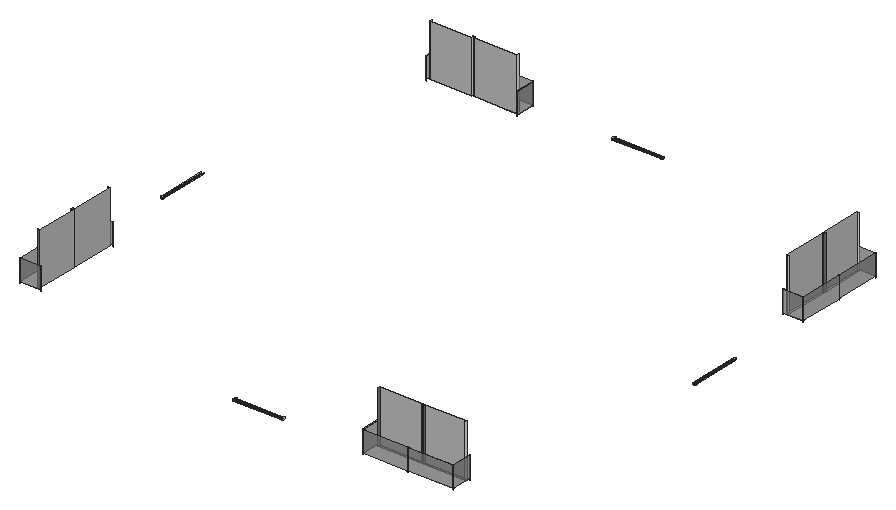
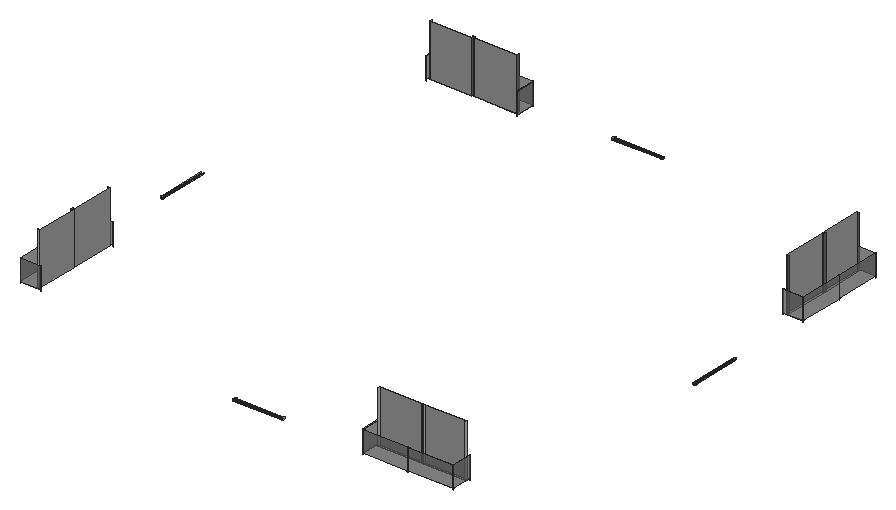
# SketchUp Ruby script. Lengths in inches.
U = 1.inch
M = Sketchup.active_model
def pt(a) = Geom::Point3d.new(a.map { |v| v * U })
def face(e, loops, mat)
  f = e.add_face(loops[0].map { |a| pt(a) })
  loops[1..].each { |l| e.add_face(l.map { |a| pt(a) }).erase! }
  f.material = f.back_material = mat if mat
  f
end
# faces: each face lists its corners as indices into pts; further lists are holes
def faces(e, pts, list, mat = nil) = list.each { |f| face(e, (f[0].is_a?(Array) ? f : [f]).map { |l| l.map { |i| pts[i] } }, mat) }
# xy, xz, yz: faces in a plane at the given z, y or x. An outline is a flat list of corners, or four numbers for a rectangle; further outlines are holes
def ring(l) = l.size == 4 ? [[l[0], l[1]], [l[2], l[1]], [l[2], l[3]], [l[0], l[3]]] : l.each_slice(2).to_a
def flat(e, list, mat, &to3) = list.each { |f| face(e, (f[0].is_a?(Array) ? f : [f]).map { |l| ring(l).map { |u, v| to3.(u, v) } }, mat) }
def xy(e, z, list, mat = nil) = flat(e, list, mat) { |x, y| [x, y, z] }
def xz(e, y, list, mat = nil) = flat(e, list, mat) { |x, z| [x, y, z] }
def yz(e, x, list, mat = nil) = flat(e, list, mat) { |y, z| [x, y, z] }
def lines(e, pts, list) = list.each { |a, b| e.add_line(pt(pts[a]), pt(pts[b])) }
# prism: a flat outline (further loops are holes) pulled along v
def prism(e, loops, v, mat = nil)
  f = face(e, loops, mat); d = Geom::Vector3d.new(v.map { |x| x * U })
  f.pushpull(f.normal.samedirection?(d) ? d.length : -d.length)
end
def box(e, o, s, mat = nil) = prism(e, [[o, [o[0] + s[0], o[1], o[2]], [o[0] + s[0], o[1] + s[1], o[2]], [o[0], o[1] + s[1], o[2]]]], [0, 0, s[2]], mat)
def at(x, y, z, deg = 0) = Geom::Transformation.translation(pt([x, y, z])) * Geom::Transformation.rotation(ORIGIN, Z_AXIS, deg.degrees)
def axes(o, x, y, z) = Geom::Transformation.new([*x, 0, *y, 0, *z, 0, *pt(o).to_a, 1])
def part(name) = M.definitions.add(name)
# library, detail: a bought-in or finely detailed component or shape, given as its bounding box
def library(name, o, s) = part(name).tap { |d| box(d.entities, o, s) }
def detail(e, o, s) = box(e.add_group.entities, o, s)
def put(e, d, t, mat = nil) = e.add_instance(d, t).tap { |i| i.material = mat if mat }
def group(e, t, mat = nil) = e.add_group.tap { |g| g.transformation = t; g.material = mat if mat }.entities
root = M.entities
M.materials.add("[Metal Seamed]").color = [118, 119, 115]
M.materials.add("[Mirror 01]").color = [185, 185, 185]
M.materials.add("[Translucent Glass Tinted]").color = [8, 201, 241]
M.materials["[Translucent Glass Tinted]"].alpha = 0.48
M.materials.add("[Translucent_Glass_Gray]").color = [128, 128, 128]
M.materials["[Translucent_Glass_Gray]"].alpha = 0.5
c1 = part("Staal sojle alta")
box(c1.entities,[0,0,0],[0.87,0.87,43.31])
c2 = part("gler")
box(c2.entities,[0,-0.71,0],[0.37,57.8,41.34],"[Translucent_Glass_Gray]")
xy(root,499.11,[[1161.2,84.8125,1285.04,90.8125],[1291.04,84.8125,1408.89,90.8125],[120,175.92,126,293.77],[120,299.77,126,423.61],[1494,1126.01,1500,1249.86],
  [1494,1255.86,1500,1373.7],[211.11,1458.8125,328.96,1464.8125],[334.96,1458.8125,458.8,1464.8125]])
xz(root,84.8125,[[1285.04,499.11,1291.04,647.61]],"[Metal Seamed]")
xz(root,90.8125,[[1161.2,499.11,1285.04,647.61],[1291.04,499.11,1408.89,647.61]],"[Mirror 01]")
xz(root,175.92,[[120,499.11,126,647.61]],"[Metal Seamed]")
xz(root,293.77,[[120,499.11,126,647.61]],"[Metal Seamed]")
xz(root,299.77,[[120,499.11,126,647.61]],"[Metal Seamed]")
xz(root,423.61,[[120,499.11,126,647.61]],"[Metal Seamed]")
xz(root,662.8,[[83.53,498.02,84.48,498.14,85.37,498.51,86.13,499.1,86.72,499.86,87.09,500.75,87.21,501.7,87.09,502.66,86.72,503.55,86.13,504.3125,85.37,504.9,84.48,505.27,83.53,505.39,82.57,505.27,81.68,504.9,80.92,504.3125,80.33,503.55,79.97,502.66,79.84,501.7,79.97,500.75,80.33,499.86,80.92,499.1,81.68,498.51,82.57,498.14]])
xz(root,886.83,[[1536.47,498.02,1535.52,498.14,1534.63,498.51,1533.87,499.1,1533.28,499.86,1532.91,500.75,1532.79,501.7,1532.91,502.66,1533.28,503.55,1533.87,504.3125,1534.63,504.9,1535.52,505.27,1536.47,505.39,1537.43,505.27,1538.32,504.9,1539.08,504.3125,1539.67,503.55,1540.03,502.66,1540.16,501.7,1540.03,500.75,1539.67,499.86,1539.08,499.1,1538.32,498.51,1537.43,498.14]])
xz(root,1126.01,[[1494,499.11,1500,647.61]])
xz(root,1249.86,[[1494,499.11,1500,647.61]])
xz(root,1255.86,[[1494,499.11,1500,647.61]])
xz(root,1373.7,[[1494,499.11,1500,647.61]])
xz(root,1458.8125,[[211.11,499.11,328.96,647.61],[334.96,499.11,458.8,647.61]],"[Mirror 01]")
xz(root,1464.8125,[[328.96,499.11,334.96,647.61]],"[Metal Seamed]")
yz(root,120,[[293.77,499.11,299.77,647.61]],"[Metal Seamed]")
yz(root,126,[[175.92,499.11,293.77,647.61],[299.77,499.11,423.61,647.61]],"[Mirror 01]")
yz(root,211.11,[[1458.8125,499.11,1464.8125,647.61]])
yz(root,328.96,[[1458.8125,499.11,1464.8125,647.61]])
yz(root,334.96,[[1458.8125,499.11,1464.8125,647.61]])
yz(root,458.8,[[1458.8125,499.11,1464.8125,647.61]])
yz(root,697.99,[[1501.28,498.02,1500.33,498.14,1499.44,498.51,1498.68,499.1,1498.09,499.86,1497.72,500.75,1497.6,501.7,1497.72,502.66,1498.09,503.55,1498.68,504.3125,1499.44,504.9,1500.33,505.27,1501.28,505.39,1502.24,505.27,1503.13,504.9,1503.89,504.3125,1504.48,503.55,1504.85,502.66,1504.97,501.7,1504.85,500.75,1504.48,499.86,1503.89,499.1,1503.13,498.51,1502.24,498.14]])
yz(root,922.01,[[48.34,498.02,49.29,498.14,50.18,498.51,50.95,499.1,51.53,499.86,51.9,500.75,52.03,501.7,51.9,502.66,51.53,503.55,50.95,504.3125,50.18,504.9,49.29,505.27,48.34,505.39,47.38,505.27,46.5,504.9,45.73,504.3125,45.15,503.55,44.78,502.66,44.65,501.7,44.78,500.75,45.15,499.86,45.73,499.1,46.5,498.51,47.38,498.14]])
yz(root,1161.2,[[84.8125,499.11,90.8125,647.61]],"[Metal Seamed]")
yz(root,1285.04,[[84.8125,499.11,90.8125,647.61]])
yz(root,1291.04,[[84.8125,499.11,90.8125,647.61]],"[Metal Seamed]")
yz(root,1408.89,[[84.8125,499.11,90.8125,647.61]])
yz(root,1494,[[1126.01,499.11,1249.86,647.61],[1255.86,499.11,1373.7,647.61]],"[Mirror 01]")
yz(root,1500,[[1249.86,499.11,1255.86,647.61]],"[Metal Seamed]")
p = [[922.01,48.34,498.02],[922.01,47.38,498.14],[778.64,47.38,498.14],[778.64,48.34,498.02],[922.01,49.29,498.14],[778.64,49.29,498.14],
  [83.53,662.8,498.02],[82.57,662.8,498.14],[82.57,806.17,498.14],[83.53,806.17,498.02],[84.48,662.8,498.14],[84.48,806.17,498.14],
  [1535.52,886.83,498.14],[1536.47,886.83,498.02],[1536.47,743.45,498.02],[1535.52,743.45,498.14],[1537.43,886.83,498.14],[1537.43,743.45,498.14],
  [697.99,1500.33,498.14],[697.99,1501.28,498.02],[841.36,1501.28,498.02],[841.36,1500.33,498.14],[697.99,1502.24,498.14],[841.36,1502.24,498.14],
  [922.01,46.5,498.51],[778.64,46.5,498.51],[922.01,50.18,498.51],[778.64,50.18,498.51],[81.68,662.8,498.51],[81.68,806.17,498.51],
  [85.37,662.8,498.51],[85.37,806.17,498.51],[1534.63,886.83,498.51],[1534.63,743.45,498.51],[1538.32,886.83,498.51],[1538.32,743.45,498.51],
  [697.99,1499.44,498.51],[841.36,1499.44,498.51],[697.99,1503.13,498.51],[841.36,1503.13,498.51],[922.01,45.73,499.1],[778.64,45.73,499.1],
  [922.01,50.95,499.1],[778.64,50.95,499.1],[80.92,662.8,499.1],[80.92,806.17,499.1],[86.13,662.8,499.1],[86.13,806.17,499.1],
  [1533.87,886.83,499.1],[1533.87,743.45,499.1],[1539.08,886.83,499.1],[1539.08,743.45,499.1],[697.99,1498.68,499.1],[841.36,1498.68,499.1],
  [697.99,1503.89,499.1],[841.36,1503.89,499.1],[922.01,45.15,499.86],[778.64,45.15,499.86],[922.01,51.53,499.86],[778.64,51.53,499.86],
  [80.33,662.8,499.86],[80.33,806.17,499.86],[86.72,662.8,499.86],[86.72,806.17,499.86],[1533.28,886.83,499.86],[1533.28,743.45,499.86],
  [1539.67,886.83,499.86],[1539.67,743.45,499.86],[697.99,1498.09,499.86],[841.36,1498.09,499.86],[697.99,1504.48,499.86],[841.36,1504.48,499.86],
  [922.01,44.78,500.75],[778.64,44.78,500.75],[922.01,51.9,500.75],[778.64,51.9,500.75],[79.97,662.8,500.75],[79.97,806.17,500.75],
  [87.09,662.8,500.75],[87.09,806.17,500.75],[1532.91,886.83,500.75],[1532.91,743.45,500.75],[1540.03,886.83,500.75],[1540.03,743.45,500.75],
  [697.99,1497.72,500.75],[841.36,1497.72,500.75],[697.99,1504.85,500.75],[841.36,1504.85,500.75],[922.01,44.65,501.7],[778.64,44.65,501.7],
  [922.01,52.03,501.7],[778.64,52.03,501.7],[79.84,662.8,501.7],[79.84,806.17,501.7],[87.21,662.8,501.7],[87.21,806.17,501.7],
  [1532.79,886.83,501.7],[1532.79,743.45,501.7],[1540.16,886.83,501.7],[1540.16,743.45,501.7],[697.99,1497.6,501.7],[841.36,1497.6,501.7],
  [697.99,1504.97,501.7],[841.36,1504.97,501.7],[922.01,44.78,502.66],[778.64,44.78,502.66],[922.01,51.9,502.66],[778.64,51.9,502.66],
  [79.97,662.8,502.66],[79.97,806.17,502.66],[87.09,662.8,502.66],[87.09,806.17,502.66],[1532.91,886.83,502.66],[1532.91,743.45,502.66],
  [1540.03,886.83,502.66],[1540.03,743.45,502.66],[697.99,1497.72,502.66],[841.36,1497.72,502.66],[697.99,1504.85,502.66],[841.36,1504.85,502.66],
  [1536.47,886.83,501.7],[1536.47,743.45,501.7],[922.01,48.34,501.7],[778.64,48.34,501.7],[697.99,1501.28,501.7],[841.36,1501.28,501.7],
  [83.53,662.8,501.7],[83.53,806.17,501.7]]
faces(root,p,[[0,1,2,3],[4,0,3,5],[6,7,8,9],[10,6,9,11],[12,13,14,15],[13,16,17,14],[18,19,20,21],[19,22,23,20],
  [1,24,25,2],[26,4,5,27],[7,28,29,8],[30,10,11,31],[32,12,15,33],[16,34,35,17],[36,18,21,37],[22,38,39,23],
  [24,40,41,25],[42,26,27,43],[28,44,45,29],[46,30,31,47],[48,32,33,49],[34,50,51,35],[52,36,37,53],[38,54,55,39],
  [40,56,57,41],[58,42,43,59],[44,60,61,45],[62,46,47,63],[64,48,49,65],[50,66,67,51],[68,52,53,69],[54,70,71,55],
  [56,72,73,57],[74,58,59,75],[60,76,77,61],[78,62,63,79],[80,64,65,81],[66,82,83,67],[84,68,69,85],[70,86,87,71],
  [72,88,89,73],[90,74,75,91],[76,92,93,77],[94,78,79,95],[96,80,81,97],[82,98,99,83],[100,84,85,101],[86,102,103,87],
  [88,104,105,89],[106,90,91,107],[92,108,109,93],[110,94,95,111],[112,96,97,113],[98,114,115,99],[116,100,101,117],[102,118,119,103]])
lines(root,p,[[120,121],[122,123],[124,125],[126,127]])
put(root,c1,axes([74.69,427.66,495.08],[0,2.19843,0],[-1,0,0],[0,0,1.5]),"[Translucent Glass Tinted]")
put(root,c1,axes([74.69,169.92,495.08],[0,2.19843,0],[-1,0,0],[0,0,1.5]),"[Translucent Glass Tinted]")
put(root,c1,axes([132.87,427.66,495.08],[0,2.19843,0],[-1,0,0],[0,0,1.5]),"[Translucent Glass Tinted]")
put(root,c1,axes([205.11,1451.94,495.08],[2.19843,0,0],[0,1,0],[0,0,1.5]),"[Translucent Glass Tinted]")
put(root,c1,axes([1414.89,97.68,495.08],[-2.19843,0,0],[0,-1,0],[0,0,1.5]),"[Translucent Glass Tinted]")
put(root,c1,axes([1545.31,1121.96,495.08],[0,-2.19843,0],[1,0,0],[0,0,1.5]),"[Translucent Glass Tinted]")
put(root,c1,axes([1414.89,39.5,495.08],[-2.19843,0,0],[0,-1,0],[0,0,1.5]),"[Translucent Glass Tinted]")
put(root,c1,axes([1157.15,97.68,495.08],[-2.19843,0,0],[0,-1,0],[0,0,1.5]),"[Translucent Glass Tinted]")
put(root,c1,axes([462.85,1510.125,495.08],[2.19843,0,0],[0,1,0],[0,0,1.5]),"[Translucent Glass Tinted]")
put(root,c1,axes([333.88,1510.125,495.08],[2.19843,0,0],[0,1,0],[0,0,1.5]),"[Translucent Glass Tinted]")
put(root,c1,axes([1487.13,1379.7,495.08],[0,-2.19843,0],[1,0,0],[0,0,1.5]),"[Translucent Glass Tinted]")
put(root,c1,axes([1487.13,1121.96,495.08],[0,-2.19843,0],[1,0,0],[0,0,1.5]),"[Translucent Glass Tinted]")
put(root,c1,axes([462.85,1451.94,495.08],[2.19843,0,0],[0,1,0],[0,0,1.5]),"[Translucent Glass Tinted]")
put(root,c1,axes([1286.12,39.5,495.08],[-2.19843,0,0],[0,-1,0],[0,0,1.5]),"[Translucent Glass Tinted]")
put(root,c1,axes([1157.15,39.5,495.08],[-2.19843,0,0],[0,-1,0],[0,0,1.5]),"[Translucent Glass Tinted]")
put(root,c1,axes([1545.31,1250.93,495.08],[0,-2.19843,0],[1,0,0],[0,0,1.5]),"[Translucent Glass Tinted]")
put(root,c1,axes([74.69,298.69,495.08],[0,2.19843,0],[-1,0,0],[0,0,1.5]),"[Translucent Glass Tinted]")
put(root,c1,axes([205.11,1510.125,495.08],[2.19843,0,0],[0,1,0],[0,0,1.5]),"[Translucent Glass Tinted]")
put(root,c1,axes([132.87,169.92,495.08],[0,2.19843,0],[-1,0,0],[0,0,1.5]),"[Translucent Glass Tinted]")
put(root,c1,axes([1545.31,1379.7,495.08],[0,-2.19843,0],[1,0,0],[0,0,1.5]),"[Translucent Glass Tinted]")
put(root,c2,axes([131.77,169.92,498.03],[0,2.19843,0],[-1,0,0],[0,0,1.5]),"[Translucent Glass Tinted]")
put(root,c2,axes([131.77,428.84,498.03],[0,2.19843,0],[-1,0,0],[0,0,1.5]),"[Translucent Glass Tinted]")
put(root,c2,axes([1411.62,38.625,498.03],[0,1,0],[-2.19843,0,0],[0,0,1.5]),"[Translucent Glass Tinted]")
put(root,c2,axes([337.35,1511,498.03],[0,-1,0],[2.19843,0,0],[0,0,1.5]),"[Translucent Glass Tinted]")
put(root,c2,axes([1414.89,96.58,498.03],[-2.19843,0,0],[0,-1,0],[0,0,1.5]),"[Translucent Glass Tinted]")
put(root,c2,axes([208.38,1511,498.03],[0,-1,0],[2.19843,0,0],[0,0,1.5]),"[Translucent Glass Tinted]")
put(root,c2,axes([464.03,1453.04,498.03],[2.19843,0,0],[0,1,0],[0,0,1.5]),"[Translucent Glass Tinted]")
put(root,c2,axes([1488.23,1120.78,498.03],[0,-2.19843,0],[1,0,0],[0,0,1.5]),"[Translucent Glass Tinted]")
put(root,c2,axes([73.81,302.16,498.03],[1,0,0],[0,2.19843,0],[0,0,1.5]),"[Translucent Glass Tinted]")
put(root,c2,axes([1282.65,38.625,498.03],[0,1,0],[-2.19843,0,0],[0,0,1.5]),"[Translucent Glass Tinted]")
put(root,c2,axes([205.11,1453.04,498.03],[2.19843,0,0],[0,1,0],[0,0,1.5]),"[Translucent Glass Tinted]")
put(root,c2,axes([1546.19,1376.43,498.03],[-1,0,0],[0,-2.19843,0],[0,0,1.5]),"[Translucent Glass Tinted]")
put(root,c2,axes([1155.97,96.58,498.03],[-2.19843,0,0],[0,-1,0],[0,0,1.5]),"[Translucent Glass Tinted]")
put(root,c2,axes([1488.23,1379.7,498.03],[0,-2.19843,0],[1,0,0],[0,0,1.5]),"[Translucent Glass Tinted]")
put(root,c2,axes([73.81,173.19,498.03],[1,0,0],[0,2.19843,0],[0,0,1.5]),"[Translucent Glass Tinted]")
put(root,c2,axes([1546.19,1247.46,498.03],[-1,0,0],[0,-2.19843,0],[0,0,1.5]),"[Translucent Glass Tinted]")
